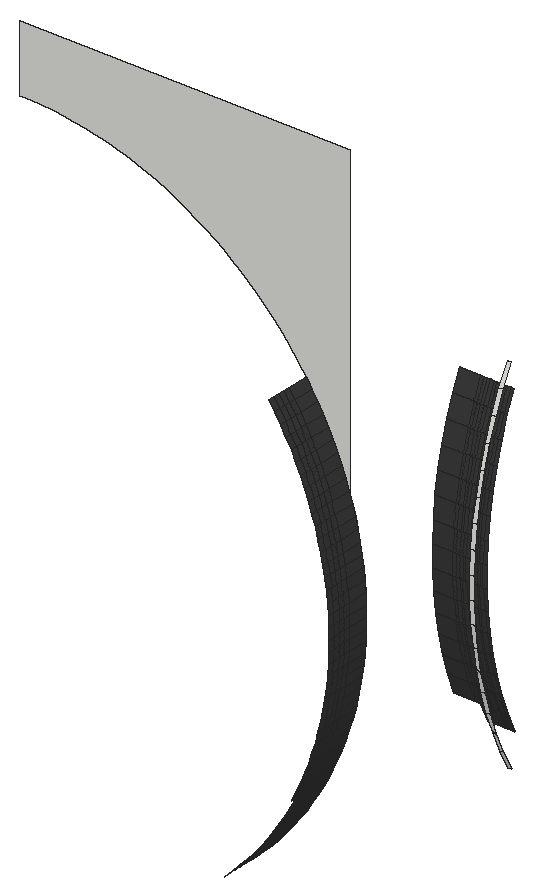
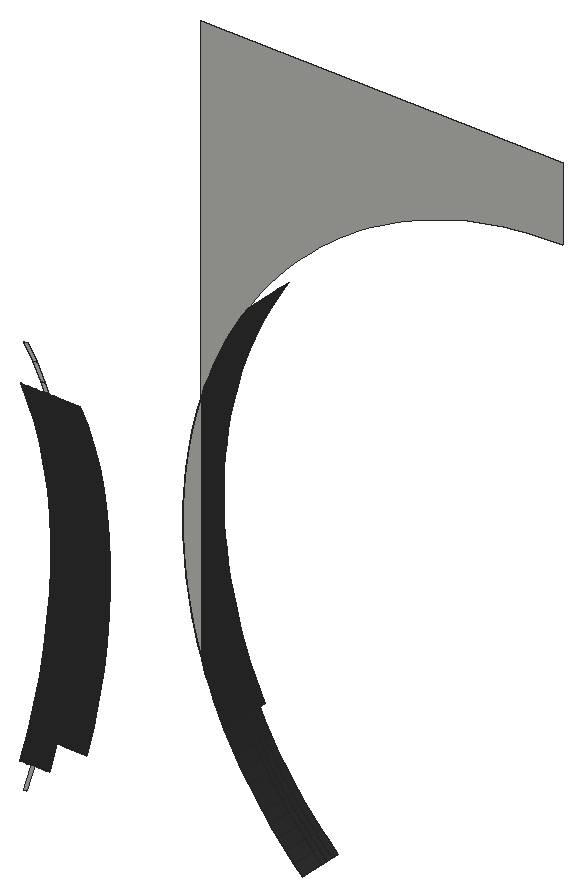
# SketchUp Ruby script. Lengths in inches.
U = 1.inch
M = Sketchup.active_model
def pt(a) = Geom::Point3d.new(a.map { |v| v * U })
def face(e, loops, mat)
  f = e.add_face(loops[0].map { |a| pt(a) })
  loops[1..].each { |l| e.add_face(l.map { |a| pt(a) }).erase! }
  f.material = f.back_material = mat if mat
  f
end
# faces: each face lists its corners as indices into pts; further lists are holes
def faces(e, pts, list, mat = nil) = list.each { |f| face(e, (f[0].is_a?(Array) ? f : [f]).map { |l| l.map { |i| pts[i] } }, mat) }
# xy, xz, yz: faces in a plane at the given z, y or x. An outline is a flat list of corners, or four numbers for a rectangle; further outlines are holes
def ring(l) = l.size == 4 ? [[l[0], l[1]], [l[2], l[1]], [l[2], l[3]], [l[0], l[3]]] : l.each_slice(2).to_a
def flat(e, list, mat, &to3) = list.each { |f| face(e, (f[0].is_a?(Array) ? f : [f]).map { |l| ring(l).map { |u, v| to3.(u, v) } }, mat) }
def xy(e, z, list, mat = nil) = flat(e, list, mat) { |x, y| [x, y, z] }
def xz(e, y, list, mat = nil) = flat(e, list, mat) { |x, z| [x, y, z] }
def yz(e, x, list, mat = nil) = flat(e, list, mat) { |y, z| [x, y, z] }
def lines(e, pts, list) = list.each { |a, b| e.add_line(pt(pts[a]), pt(pts[b])) }
# prism: a flat outline (further loops are holes) pulled along v
def prism(e, loops, v, mat = nil)
  f = face(e, loops, mat); d = Geom::Vector3d.new(v.map { |x| x * U })
  f.pushpull(f.normal.samedirection?(d) ? d.length : -d.length)
end
def box(e, o, s, mat = nil) = prism(e, [[o, [o[0] + s[0], o[1], o[2]], [o[0] + s[0], o[1] + s[1], o[2]], [o[0], o[1] + s[1], o[2]]]], [0, 0, s[2]], mat)
def at(x, y, z, deg = 0) = Geom::Transformation.translation(pt([x, y, z])) * Geom::Transformation.rotation(ORIGIN, Z_AXIS, deg.degrees)
def axes(o, x, y, z) = Geom::Transformation.new([*x, 0, *y, 0, *z, 0, *pt(o).to_a, 1])
def part(name) = M.definitions.add(name)
# library, detail: a bought-in or finely detailed component or shape, given as its bounding box
def library(name, o, s) = part(name).tap { |d| box(d.entities, o, s) }
def detail(e, o, s) = box(e.add_group.entities, o, s)
def put(e, d, t, mat = nil) = e.add_instance(d, t).tap { |i| i.material = mat if mat }
def group(e, t, mat = nil) = e.add_group.tap { |g| g.transformation = t; g.material = mat if mat }.entities
root = M.entities
M.materials.add("[Color M07]").color = [58, 58, 58]
xz(root,124.96,[[190.96,280.4375,191.22,281.29,191.54,282.45,191.82,283.62,192.0625,284.8,192.27,285.98,192.44,287.17,192.57,288.37,192.67,289.57,192.72,290.77,192.74,291.97,192.72,293.17,192.67,294.37,192.57,295.57,192.44,296.77,192.27,297.96,192.0625,299.14,191.82,300.32,191.54,301.49,191.22,302.65,190.96,303.5],[190.96,303.5,190.87,303.8,190.48,304.9375,190.05,306.0625,189.59,307.17,189.1,308.27,188.57,309.35,188.01,310.41,187.41,311.46,186.78,312.48,186.12,313.49,185.43,314.47,184.71,315.43,183.96,316.37,183.18,317.28,182.37,318.17,181.53,319.04,180.67,319.875,179.78,320.68,178.86,321.46,177.92,322.22,176.96,322.9375,175.98,323.63,174.97,324.29,173.95,324.92,172.9,325.51,171.84,326.08,170.76,326.61,169.66,327.1,168.55,327.5625,167.43,327.99,166.29,328.375,165.14,328.73,163.98,329.05,162.8125,329.33,161.63,329.57,160.45,329.78,159.26,329.95,158.0625,330.08,156.86,330.17,155.66,330.23,154.46,330.25,154.46,337.6875,190.96,337.6875]])
xz(root,136.33,[[190.96,291.31,193.21,293.66],[193.21,291.31,193.59,293.66],[193.59,291.31,193.96,293.66],[193.96,291.31,194.34,293.66],[194.34,291.31,194.71,293.66],
  [194.71,291.31,195.09,293.66],[195.09,291.31,195.46,293.66],[195.46,291.31,195.84,293.66],[195.84,291.31,196.21,293.66],[196.21,291.31,196.59,293.66],
  [196.59,291.31,196.96,293.66]],"[Color M07]")
p = [[181.53,120.52,264.9],[181.53,121.21,264.9],[180.67,121.21,264.0625],[180.67,120.52,264.0625],[181.53,121.89,264.9],[180.67,121.89,264.0625],
  [181.53,122.58,264.9],[180.67,122.58,264.0625],[180.67,124.96,264.0625],[181.53,124.96,264.9],[182.37,120.52,265.76],[182.37,121.21,265.76],
  [182.37,121.89,265.76],[182.37,122.58,265.76],[182.37,124.96,265.76],[183.18,120.52,266.65],[183.18,121.21,266.65],[183.18,121.89,266.65],
  [183.18,122.58,266.65],[183.18,124.96,266.65],[183.96,120.52,267.57],[183.96,121.21,267.57],[183.96,121.89,267.57],[183.96,122.58,267.57],
  [183.96,124.96,267.57],[184.71,120.52,268.51],[184.71,121.21,268.51],[184.71,121.89,268.51],[184.71,122.58,268.51],[184.71,124.96,268.51],
  [185.43,120.52,269.47],[185.43,121.21,269.47],[185.43,121.89,269.47],[185.43,122.58,269.47],[185.43,124.96,269.47],[186.12,120.52,270.45],
  [186.12,121.21,270.45],[186.12,121.89,270.45],[186.12,122.58,270.45],[186.12,124.96,270.45],[186.78,120.52,271.46],[186.78,121.21,271.46],
  [186.78,121.89,271.46],[186.78,122.58,271.46],[186.78,124.96,271.46],[187.41,120.52,272.48],[187.41,121.21,272.48],[187.41,121.89,272.48],
  [187.41,122.58,272.48],[187.41,124.96,272.48],[196.96,139.28,272.3],[196.96,138.14,274.5],[197.34,138.14,274.5],[197.34,139.28,272.3],
  [188.01,120.52,273.53],[188.01,121.21,273.53],[188.01,121.89,273.53],[188.01,122.58,273.53],[188.01,124.96,273.53],[188.57,120.52,274.59],
  [188.57,121.21,274.59],[188.57,121.89,274.59],[188.57,122.58,274.59],[188.57,124.96,274.59],[196.96,137.14,276.77],[197.34,137.14,276.77],
  [189.1,119.83,275.67],[189.1,120.52,275.67],[188.57,119.83,274.59],[189.1,121.21,275.67],[189.1,121.89,275.67],[189.1,122.58,275.67],
  [189.1,124.96,275.67],[194.34,140.2,275.49],[193.96,140.2,275.49],[193.96,139.25,277.63],[194.34,139.25,277.63],[194.71,140.2,275.49],
  [194.71,139.25,277.63],[195.09,140.2,275.49],[195.09,139.25,277.63],[195.46,140.2,275.49],[195.46,139.25,277.63],[195.84,140.2,275.49],
  [195.84,139.25,277.63],[196.21,140.2,275.49],[196.21,139.25,277.63],[196.59,140.2,275.49],[196.59,139.25,277.63],[196.96,140.2,275.49],
  [196.96,139.25,277.63],[189.59,119.83,276.77],[189.59,120.52,276.77],[189.59,121.21,276.77],[189.59,121.89,276.77],[189.59,122.58,276.77],
  [189.59,124.96,276.77],[190.05,119.83,277.875],[190.05,120.52,277.875],[190.05,121.21,277.875],[190.05,121.89,277.875],[190.05,122.58,277.875],
  [190.05,124.96,277.875],[196.96,136.27,279.09],[197.34,136.27,279.09],[190.96,138.43,279.83],[193.21,138.43,279.83],[193.21,139.25,277.63],
  [190.96,139.25,277.63],[193.59,139.25,277.63],[193.59,138.43,279.83],[193.96,138.43,279.83],[194.34,138.43,279.83],[194.71,138.43,279.83],
  [195.09,138.43,279.83],[195.46,138.43,279.83],[195.84,138.43,279.83],[196.21,138.43,279.83],[196.59,138.43,279.83],[196.96,138.43,279.83],
  [190.48,119.83,279],[190.48,120.52,279],[190.48,121.21,279],[190.48,121.89,279],[190.48,122.58,279],[190.48,124.96,279],
  [190.87,119.83,280.14],[190.87,120.52,280.14],[190.87,121.21,280.14],[190.87,121.89,280.14],[190.87,122.58,280.14],[190.87,124.96,280.14],
  [196.96,135.54,281.46],[197.34,135.54,281.46],[190.96,137.74,282.07],[193.21,137.74,282.07],[193.59,137.74,282.07],[193.96,137.74,282.07],
  [194.34,137.74,282.07],[194.71,137.74,282.07],[195.09,137.74,282.07],[195.46,137.74,282.07],[195.84,137.74,282.07],[196.21,137.74,282.07],
  [196.59,137.74,282.07],[196.96,137.74,282.07],[191.22,119.83,281.29],[191.22,120.52,281.29],[191.22,121.21,281.29],[191.22,121.89,281.29],
  [191.22,122.58,281.29],[191.22,124.96,281.29],[190.96,124.96,280.4375],[191.54,119.83,282.45],[191.54,120.52,282.45],[191.54,121.21,282.45],
  [191.54,121.89,282.45],[191.54,122.58,282.45],[191.54,124.96,282.45],[196.96,134.95,283.87],[197.34,134.95,283.87],[190.96,137.18,284.34],
  [193.21,137.18,284.34],[193.59,137.18,284.34],[193.96,137.18,284.34],[194.34,137.18,284.34],[194.71,137.18,284.34],[195.09,137.18,284.34],
  [195.46,137.18,284.34],[195.84,137.18,284.34],[196.21,137.18,284.34],[196.59,137.18,284.34],[196.96,137.18,284.34],[191.82,119.83,283.62],
  [191.82,120.52,283.62],[191.82,121.21,283.62],[191.82,121.89,283.62],[191.82,122.58,283.62],[191.82,124.96,283.62],[192.0625,119.83,284.8],
  [192.0625,120.52,284.8],[192.0625,121.21,284.8],[192.0625,121.89,284.8],[192.0625,122.58,284.8],[192.0625,124.96,284.8],[196.96,134.5,286.31],
  [197.34,134.5,286.31],[190.96,136.76,286.65],[193.21,136.76,286.65],[193.59,136.76,286.65],[193.96,136.76,286.65],[194.34,136.76,286.65],
  [194.71,136.76,286.65],[195.09,136.76,286.65],[195.46,136.76,286.65],[195.84,136.76,286.65],[196.21,136.76,286.65],[196.59,136.76,286.65],
  [196.96,136.76,286.65],[192.27,119.83,285.98],[192.27,120.52,285.98],[192.27,121.21,285.98],[192.27,121.89,285.98],[192.27,122.58,285.98],
  [192.27,124.96,285.98],[192.44,119.83,287.17],[192.44,120.52,287.17],[192.44,121.21,287.17],[192.44,121.89,287.17],[192.44,122.58,287.17],
  [192.44,124.96,287.17],[196.96,134.2,288.77],[197.34,134.2,288.77],[190.96,136.48,288.98],[193.21,136.48,288.98],[193.59,136.48,288.98],
  [193.96,136.48,288.98],[194.34,136.48,288.98],[194.71,136.48,288.98],[195.09,136.48,288.98],[195.46,136.48,288.98],[195.84,136.48,288.98],
  [196.21,136.48,288.98],[196.59,136.48,288.98],[196.96,136.48,288.98],[192.57,119.83,288.37],[192.57,120.52,288.37],[192.57,121.21,288.37],
  [192.57,121.89,288.37],[192.57,122.58,288.37],[192.57,124.96,288.37],[192.67,119.83,289.57],[192.67,120.52,289.57],[192.67,121.21,289.57],
  [192.67,121.89,289.57],[192.67,122.58,289.57],[192.67,124.96,289.57],[196.96,134.05,291.24],[197.34,134.05,291.24],[190.96,136.33,291.31],
  [193.21,136.33,291.31],[193.59,136.33,291.31],[193.96,136.33,291.31],[194.34,136.33,291.31],[194.71,136.33,291.31],[195.09,136.33,291.31],
  [195.46,136.33,291.31],[195.84,136.33,291.31],[196.21,136.33,291.31],[196.59,136.33,291.31],[196.96,136.33,291.31],[192.72,119.83,290.77],
  [192.72,120.52,290.77],[192.72,121.21,290.77],[192.72,121.89,290.77],[192.72,122.58,290.77],[192.72,124.96,290.77],[192.74,119.83,291.97],
  [192.74,120.52,291.97],[192.74,121.21,291.97],[192.74,121.89,291.97],[192.74,122.58,291.97],[192.74,124.96,291.97],[196.96,134.04,293.72],
  [197.34,134.04,293.72],[192.72,119.83,293.17],[192.72,120.52,293.17],[192.72,121.21,293.17],[192.72,121.89,293.17],[192.72,122.58,293.17],
  [192.72,124.96,293.17],[192.67,119.83,294.37],[192.67,120.52,294.37],[192.67,121.21,294.37],[192.67,121.89,294.37],[192.67,122.58,294.37],
  [192.67,124.96,294.37],[196.96,134.1875,296.2],[197.34,134.1875,296.2],[190.96,136.46,296],[193.21,136.46,296],[193.21,136.33,293.66],
  [190.96,136.33,293.66],[193.59,136.33,293.66],[193.59,136.46,296],[193.96,136.33,293.66],[193.96,136.46,296],[194.34,136.33,293.66],
  [194.34,136.46,296],[194.71,136.33,293.66],[194.71,136.46,296],[195.09,136.33,293.66],[195.09,136.46,296],[195.46,136.33,293.66],
  [195.46,136.46,296],[195.84,136.33,293.66],[195.84,136.46,296],[196.21,136.33,293.66],[196.21,136.46,296],[196.59,136.33,293.66],
  [196.59,136.46,296],[196.96,136.33,293.66],[196.96,136.46,296],[192.57,119.83,295.57],[192.57,120.52,295.57],[192.57,121.21,295.57],
  [192.57,121.89,295.57],[192.57,122.58,295.57],[192.57,124.96,295.57],[192.44,119.83,296.77],[192.44,120.52,296.77],[192.44,121.21,296.77],
  [192.44,121.89,296.77],[192.44,122.58,296.77],[192.44,124.96,296.77],[190.96,136.73,298.33],[193.21,136.73,298.33],[193.59,136.73,298.33],
  [193.96,136.73,298.33],[194.34,136.73,298.33],[194.71,136.73,298.33],[195.09,136.73,298.33],[195.46,136.73,298.33],[195.84,136.73,298.33],
  [196.21,136.73,298.33],[196.59,136.73,298.33],[196.96,136.73,298.33],[196.96,134.47,298.66],[197.34,134.47,298.66],[192.27,119.83,297.96],
  [192.27,120.52,297.96],[192.27,121.21,297.96],[192.27,121.89,297.96],[192.27,122.58,297.96],[192.27,124.96,297.96],[192.0625,119.83,299.14],
  [192.0625,120.52,299.14],[192.0625,121.21,299.14],[192.0625,121.89,299.14],[192.0625,122.58,299.14],[192.0625,124.96,299.14],[190.96,137.14,300.63],
  [193.21,137.14,300.63],[193.59,137.14,300.63],[193.96,137.14,300.63],[194.34,137.14,300.63],[194.71,137.14,300.63],[195.09,137.14,300.63],
  [195.46,137.14,300.63],[195.84,137.14,300.63],[196.21,137.14,300.63],[196.59,137.14,300.63],[196.96,137.14,300.63],[196.96,134.91,301.1],
  [197.34,134.91,301.1],[191.82,119.83,300.32],[191.82,120.52,300.32],[191.82,121.21,300.32],[191.82,121.89,300.32],[191.82,122.58,300.32],
  [191.82,124.96,300.32],[191.54,119.83,301.49],[191.54,120.52,301.49],[191.54,121.21,301.49],[191.54,121.89,301.49],[191.54,122.58,301.49],
  [191.54,124.96,301.49],[190.96,137.6875,302.91],[193.21,137.6875,302.91],[193.59,137.6875,302.91],[193.96,137.6875,302.91],[194.34,137.6875,302.91],
  [194.71,137.6875,302.91],[195.09,137.6875,302.91],[195.46,137.6875,302.91],[195.84,137.6875,302.91],[196.21,137.6875,302.91],[196.59,137.6875,302.91],
  [196.96,137.6875,302.91],[196.96,135.48,303.51],[197.34,135.48,303.51],[191.22,119.83,302.65],[191.22,120.52,302.65],[191.22,121.21,302.65],
  [191.22,121.89,302.65],[191.22,122.58,302.65],[191.22,124.96,302.65],[190.87,119.83,303.8],[190.87,120.52,303.8],[190.87,121.21,303.8],
  [190.87,121.89,303.8],[190.87,122.58,303.8],[190.87,124.96,303.8],[190.96,124.96,303.5],[190.96,138.37,305.15],[193.21,138.37,305.15],
  [193.59,138.37,305.15],[193.96,138.37,305.15],[194.34,138.37,305.15],[194.71,138.37,305.15],[195.09,138.37,305.15],[195.46,138.37,305.15],
  [195.84,138.37,305.15],[196.21,138.37,305.15],[196.59,138.37,305.15],[196.96,138.37,305.15],[196.96,136.2,305.88],[197.34,136.2,305.88],
  [190.48,119.83,304.9375],[190.48,120.52,304.9375],[190.48,121.21,304.9375],[190.48,121.89,304.9375],[190.48,122.58,304.9375],[190.48,124.96,304.9375],
  [190.05,119.83,306.0625],[190.05,120.52,306.0625],[190.05,121.21,306.0625],[190.05,121.89,306.0625],[190.05,122.58,306.0625],[190.05,124.96,306.0625],
  [190.96,139.18,307.35],[193.21,139.18,307.35],[193.59,139.18,307.35],[193.96,139.18,307.35],[194.34,139.18,307.35],[194.71,139.18,307.35],
  [195.09,139.18,307.35],[195.46,139.18,307.35],[195.84,139.18,307.35],[196.21,139.18,307.35],[196.59,139.18,307.35],[196.96,139.18,307.35],
  [196.96,137.0625,308.21],[197.34,137.0625,308.21],[189.59,119.83,307.17],[189.59,120.52,307.17],[189.59,121.21,307.17],[189.59,121.89,307.17],
  [189.59,122.58,307.17],[189.59,124.96,307.17],[189.1,119.83,308.27],[189.1,120.52,308.27],[189.1,121.21,308.27],[189.1,121.89,308.27],
  [189.1,122.58,308.27],[189.1,124.96,308.27],[190.96,140.12,309.5],[193.21,140.12,309.5],[193.59,140.12,309.5],[193.96,140.12,309.5],
  [194.34,140.12,309.5],[194.71,140.12,309.5],[195.09,140.12,309.5],[195.46,140.12,309.5],[195.84,140.12,309.5],[196.21,140.12,309.5],
  [196.59,140.12,309.5],[196.96,140.12,309.5],[196.96,138.06,310.48],[197.34,138.06,310.48],[188.57,119.83,309.35],[188.57,120.52,309.35],
  [188.57,121.21,309.35],[188.57,121.89,309.35],[188.57,122.58,309.35],[188.57,124.96,309.35],[188.01,119.83,310.41],[188.01,120.52,310.41],
  [188.01,121.21,310.41],[188.01,121.89,310.41],[188.01,122.58,310.41],[188.01,124.96,310.41],[187.41,119.83,311.46],[187.41,120.52,311.46],
  [187.41,121.21,311.46],[187.41,121.89,311.46],[187.41,122.58,311.46],[187.41,124.96,311.46],[196.96,139.1875,312.6875],[197.34,139.1875,312.6875],
  [186.78,119.83,312.48],[186.78,120.52,312.48],[186.78,121.21,312.48],[186.78,121.89,312.48],[186.78,122.58,312.48],[186.78,124.96,312.48],
  [186.12,119.83,313.49],[186.12,120.52,313.49],[186.12,121.21,313.49],[186.12,121.89,313.49],[186.12,122.58,313.49],[186.12,124.96,313.49]]
faces(root,p,[[0,1,2,3],[1,4,5,2],[4,6,7,5],[8,7,6,9],[10,11,1,0],[11,12,4,1],[12,13,6,4],[9,6,13,14],
  [15,16,11,10],[16,17,12,11],[17,18,13,12],[14,13,18,19],[20,21,16,15],[21,22,17,16],[22,23,18,17],[19,18,23,24],
  [25,26,21,20],[26,27,22,21],[27,28,23,22],[24,23,28,29],[30,31,26,25],[31,32,27,26],[32,33,28,27],[29,28,33,34],
  [35,36,31,30],[36,37,32,31],[37,38,33,32],[34,33,38,39],[40,41,36,35],[41,42,37,36],[42,43,38,37],[39,38,43,44],
  [45,46,41,40],[46,47,42,41],[47,48,43,42],[44,43,48,49],[54,55,46,45],[55,56,47,46],[56,57,48,47],[49,48,57,58],
  [59,60,55,54],[60,61,56,55],[61,62,57,56],[58,57,62,63],[66,67,59,68],[67,69,60,59],[69,70,61,60],[70,71,62,61],
  [63,62,71,72],[73,74,75,76],[77,73,76,78],[79,77,78,80],[81,79,80,82],[83,81,82,84],[85,83,84,86],[87,85,86,88],
  [89,87,88,90],[91,92,67,66],[92,93,69,67],[93,94,70,69],[94,95,71,70],[72,71,95,96],[97,98,92,91],[98,99,93,92],
  [99,100,94,93],[100,101,95,94],[96,95,101,102],[105,106,107,108],[109,107,106,110],[75,109,110,111],[76,75,111,112],[78,76,112,113],
  [80,78,113,114],[82,80,114,115],[84,82,115,116],[86,84,116,117],[88,86,117,118],[90,88,118,119],[120,121,98,97],[121,122,99,98],
  [122,123,100,99],[123,124,101,100],[102,101,124,125],[126,127,121,120],[127,128,122,121],[128,129,123,122],[129,130,124,123],[125,124,130,131],
  [134,135,106,105],[110,106,135,136],[111,110,136,137],[112,111,137,138],[113,112,138,139],[114,113,139,140],[115,114,140,141],[116,115,141,142],
  [117,116,142,143],[118,117,143,144],[119,118,144,145],[146,147,127,126],[147,148,128,127],[148,149,129,128],[149,150,130,129],[131,130,150,151,152],
  [153,154,147,146],[154,155,148,147],[155,156,149,148],[156,157,150,149],[151,150,157,158],[161,162,135,134],[136,135,162,163],[137,136,163,164],
  [138,137,164,165],[139,138,165,166],[140,139,166,167],[141,140,167,168],[142,141,168,169],[143,142,169,170],[144,143,170,171],[145,144,171,172],
  [173,174,154,153],[174,175,155,154],[175,176,156,155],[176,177,157,156],[158,157,177,178],[179,180,174,173],[180,181,175,174],[181,182,176,175],
  [182,183,177,176],[178,177,183,184],[187,188,162,161],[163,162,188,189],[164,163,189,190],[165,164,190,191],[166,165,191,192],[167,166,192,193],
  [168,167,193,194],[169,168,194,195],[170,169,195,196],[171,170,196,197],[172,171,197,198],[199,200,180,179],[200,201,181,180],[201,202,182,181],
  [202,203,183,182],[184,183,203,204],[205,206,200,199],[206,207,201,200],[207,208,202,201],[208,209,203,202],[204,203,209,210],[213,214,188,187],
  [189,188,214,215],[190,189,215,216],[191,190,216,217],[192,191,217,218],[193,192,218,219],[194,193,219,220],[195,194,220,221],[196,195,221,222],
  [197,196,222,223],[198,197,223,224],[225,226,206,205],[226,227,207,206],[227,228,208,207],[228,229,209,208],[210,209,229,230],[231,232,226,225],
  [232,233,227,226],[233,234,228,227],[234,235,229,228],[230,229,235,236],[239,240,214,213],[215,214,240,241],[216,215,241,242],[217,216,242,243],
  [218,217,243,244],[219,218,244,245],[220,219,245,246],[221,220,246,247],[222,221,247,248],[223,222,248,249],[224,223,249,250],[251,252,232,231],
  [252,253,233,232],[253,254,234,233],[254,255,235,234],[236,235,255,256],[257,258,252,251],[258,259,253,252],[259,260,254,253],[260,261,255,254],
  [256,255,261,262],[265,266,258,257],[266,267,259,258],[267,268,260,259],[268,269,261,260],[262,261,269,270],[271,272,266,265],[272,273,267,266],
  [273,274,268,267],[274,275,269,268],[270,269,275,276],[279,280,281,282],[283,281,280,284],[285,283,284,286],[287,285,286,288],[289,287,288,290],
  [291,289,290,292],[293,291,292,294],[295,293,294,296],[297,295,296,298],[299,297,298,300],[301,299,300,302],[303,304,272,271],[304,305,273,272],
  [305,306,274,273],[306,307,275,274],[276,275,307,308],[309,310,304,303],[310,311,305,304],[311,312,306,305],[312,313,307,306],[308,307,313,314],
  [315,316,280,279],[284,280,316,317],[286,284,317,318],[288,286,318,319],[290,288,319,320],[292,290,320,321],[294,292,321,322],[296,294,322,323],
  [298,296,323,324],[300,298,324,325],[302,300,325,326],[329,330,310,309],[330,331,311,310],[331,332,312,311],[332,333,313,312],[314,313,333,334],
  [335,336,330,329],[336,337,331,330],[337,338,332,331],[338,339,333,332],[334,333,339,340],[341,342,316,315],[317,316,342,343],[318,317,343,344],
  [319,318,344,345],[320,319,345,346],[321,320,346,347],[322,321,347,348],[323,322,348,349],[324,323,349,350],[325,324,350,351],[326,325,351,352],
  [355,356,336,335],[356,357,337,336],[357,358,338,337],[358,359,339,338],[340,339,359,360],[361,362,356,355],[362,363,357,356],[363,364,358,357],
  [364,365,359,358],[360,359,365,366],[367,368,342,341],[343,342,368,369],[344,343,369,370],[345,344,370,371],[346,345,371,372],[347,346,372,373],
  [348,347,373,374],[349,348,374,375],[350,349,375,376],[351,350,376,377],[352,351,377,378],[381,382,362,361],[382,383,363,362],[383,384,364,363],
  [384,385,365,364],[366,365,385,386],[387,388,382,381],[388,389,383,382],[389,390,384,383],[390,391,385,384],[386,385,391,392,393],[394,395,368,367],
  [369,368,395,396],[370,369,396,397],[371,370,397,398],[372,371,398,399],[373,372,399,400],[374,373,400,401],[375,374,401,402],[376,375,402,403],
  [377,376,403,404],[378,377,404,405],[408,409,388,387],[409,410,389,388],[410,411,390,389],[411,412,391,390],[392,391,412,413],[414,415,409,408],
  [415,416,410,409],[416,417,411,410],[417,418,412,411],[413,412,418,419],[420,421,395,394],[396,395,421,422],[397,396,422,423],[398,397,423,424],
  [399,398,424,425],[400,399,425,426],[401,400,426,427],[402,401,427,428],[403,402,428,429],[404,403,429,430],[405,404,430,431],[434,435,415,414],
  [435,436,416,415],[436,437,417,416],[437,438,418,417],[419,418,438,439],[440,441,435,434],[441,442,436,435],[442,443,437,436],[443,444,438,437],
  [439,438,444,445],[446,447,421,420],[422,421,447,448],[423,422,448,449],[424,423,449,450],[425,424,450,451],[426,425,451,452],[427,426,452,453],
  [428,427,453,454],[429,428,454,455],[430,429,455,456],[431,430,456,457],[460,461,441,440],[461,462,442,441],[462,463,443,442],[463,464,444,443],
  [445,444,464,465],[466,467,461,460],[467,468,462,461],[468,469,463,462],[469,470,464,463],[465,464,470,471],[472,473,467,466],[473,474,468,467],
  [474,475,469,468],[475,476,470,469],[471,470,476,477],[480,481,473,472],[481,482,474,473],[482,483,475,474],[483,484,476,475],[477,476,484,485],
  [486,487,481,480],[487,488,482,481],[488,489,483,482],[489,490,484,483],[485,484,490,491]],"[Color M07]")
faces(root,p,[[50,51,52,53],[51,64,65,52],[64,103,104,65],[103,132,133,104],[132,159,160,133],[159,185,186,160],[185,211,212,186],[211,237,238,212],
  [237,263,264,238],[263,277,278,264],[277,327,328,278],[327,353,354,328],[353,379,380,354],[379,406,407,380],[406,432,433,407],[432,458,459,433],
  [458,478,479,459]])
